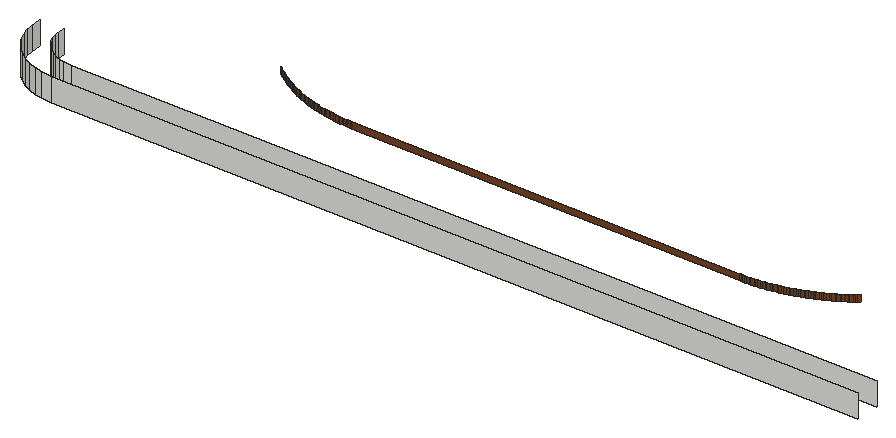
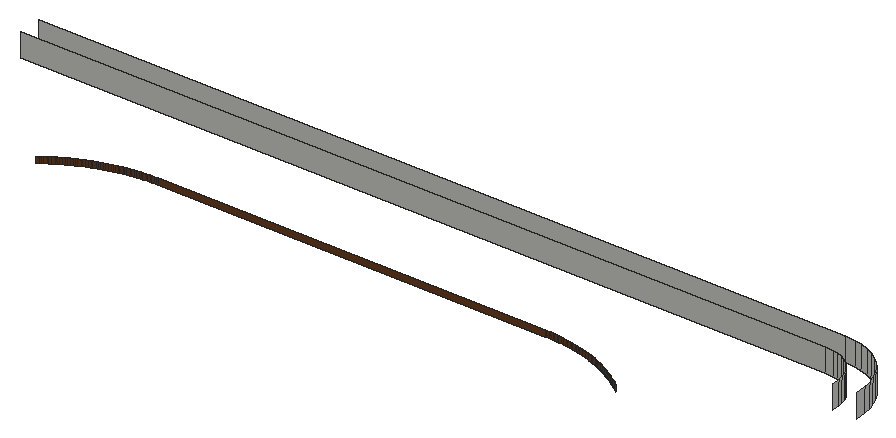
# SketchUp Ruby script. Lengths in inches.
U = 1.inch
M = Sketchup.active_model
def pt(a) = Geom::Point3d.new(a.map { |v| v * U })
def face(e, loops, mat)
  f = e.add_face(loops[0].map { |a| pt(a) })
  loops[1..].each { |l| e.add_face(l.map { |a| pt(a) }).erase! }
  f.material = f.back_material = mat if mat
  f
end
# faces: each face lists its corners as indices into pts; further lists are holes
def faces(e, pts, list, mat = nil) = list.each { |f| face(e, (f[0].is_a?(Array) ? f : [f]).map { |l| l.map { |i| pts[i] } }, mat) }
# xy, xz, yz: faces in a plane at the given z, y or x. An outline is a flat list of corners, or four numbers for a rectangle; further outlines are holes
def ring(l) = l.size == 4 ? [[l[0], l[1]], [l[2], l[1]], [l[2], l[3]], [l[0], l[3]]] : l.each_slice(2).to_a
def flat(e, list, mat, &to3) = list.each { |f| face(e, (f[0].is_a?(Array) ? f : [f]).map { |l| ring(l).map { |u, v| to3.(u, v) } }, mat) }
def xy(e, z, list, mat = nil) = flat(e, list, mat) { |x, y| [x, y, z] }
def xz(e, y, list, mat = nil) = flat(e, list, mat) { |x, z| [x, y, z] }
def yz(e, x, list, mat = nil) = flat(e, list, mat) { |y, z| [x, y, z] }
def lines(e, pts, list) = list.each { |a, b| e.add_line(pt(pts[a]), pt(pts[b])) }
# prism: a flat outline (further loops are holes) pulled along v
def prism(e, loops, v, mat = nil)
  f = face(e, loops, mat); d = Geom::Vector3d.new(v.map { |x| x * U })
  f.pushpull(f.normal.samedirection?(d) ? d.length : -d.length)
end
def box(e, o, s, mat = nil) = prism(e, [[o, [o[0] + s[0], o[1], o[2]], [o[0] + s[0], o[1] + s[1], o[2]], [o[0], o[1] + s[1], o[2]]]], [0, 0, s[2]], mat)
def at(x, y, z, deg = 0) = Geom::Transformation.translation(pt([x, y, z])) * Geom::Transformation.rotation(ORIGIN, Z_AXIS, deg.degrees)
def axes(o, x, y, z) = Geom::Transformation.new([*x, 0, *y, 0, *z, 0, *pt(o).to_a, 1])
def part(name) = M.definitions.add(name)
# library, detail: a bought-in or finely detailed component or shape, given as its bounding box
def library(name, o, s) = part(name).tap { |d| box(d.entities, o, s) }
def detail(e, o, s) = box(e.add_group.entities, o, s)
def put(e, d, t, mat = nil) = e.add_instance(d, t).tap { |i| i.material = mat if mat }
def group(e, t, mat = nil) = e.add_group.tap { |g| g.transformation = t; g.material = mat if mat }.entities
root = M.entities
M.materials.add("[Wood Veneer 01]3").color = [120, 70, 37]
xz(root,33.75,[[75.22,121,143.98,123]])
xz(root,35.75,[[75.29,121,143.97,123]])
xz(root,43.5,[[92.65,121,92.82,121.5],[92.82,121,93,121.5],[93,121,126,121.5],[126,121,126.18,121.5],[126.18,121,126.35,121.5]],"[Wood Veneer 01]3")
p = [[73.64,33.94,121],[74.32,33.81,121],[74.32,33.81,123],[73.64,33.94,123],[75.22,33.75,121],[75.22,33.75,123],
  [73,34.16,121],[73,34.16,123],[72.38,34.47,121],[72.38,34.47,123],[71.8125,34.85,121],[71.8125,34.85,123],
  [71.3,35.3,121],[71.3,35.3,123],[70.85,35.8125,121],[70.85,35.8125,123],[70.47,36.38,121],[70.47,36.38,123],
  [74.58,35.8,121],[74.16,35.88,121],[74.16,35.88,123],[74.58,35.8,123],[75.29,35.75,121],[75.29,35.75,123],
  [73.76,36.01,121],[73.76,36.01,123],[73.38,36.2,121],[73.38,36.2,123],[73.03,36.4375,121],[73.03,36.4375,123],
  [70.16,37,121],[70.16,37,123],[72.72,36.72,121],[72.72,36.72,123],[72.4375,37.03,121],[72.4375,37.03,123],
  [69.94,37.64,121],[69.94,37.64,123],[72.2,37.38,121],[72.2,37.38,123],[72.01,37.76,121],[72.01,37.76,123],
  [69.81,38.32,121],[69.81,38.32,123],[71.88,38.16,121],[71.88,38.16,123],[71.8,38.58,121],[71.8,38.58,123],
  [69.75,39.22,121],[69.75,39.22,123],[71.75,39.29,121],[71.75,39.29,123],[91.76,43.56,121],[91.94,43.54,121],
  [91.94,43.54,121.5],[91.76,43.56,121.5],[92.12,43.53,121],[92.12,43.53,121.5],[92.29,43.52,121],[92.29,43.52,121.5],
  [92.47,43.51,121],[92.47,43.51,121.5],[92.65,43.5,121],[92.65,43.5,121.5],[126.35,43.5,121],[126.53,43.51,121],
  [126.53,43.51,121.5],[126.35,43.5,121.5],[126.71,43.52,121],[126.71,43.52,121.5],[126.88,43.53,121],[126.88,43.53,121.5],
  [127.06,43.54,121],[127.06,43.54,121.5],[127.24,43.56,121],[127.24,43.56,121.5],[90.89,43.67,121],[91.0625,43.64,121],
  [91.0625,43.64,121.5],[90.89,43.67,121.5],[91.24,43.62,121],[91.24,43.62,121.5],[91.41,43.59,121],[91.41,43.59,121.5],
  [91.59,43.57,121],[91.59,43.57,121.5],[127.41,43.57,121],[127.41,43.57,121.5],[127.59,43.59,121],[127.59,43.59,121.5],
  [127.76,43.62,121],[127.76,43.62,121.5],[127.9375,43.64,121],[127.9375,43.64,121.5],[128.11,43.67,121],[128.11,43.67,121.5],
  [90.37,43.76,121],[90.54,43.73,121],[90.54,43.73,121.5],[90.37,43.76,121.5],[90.71,43.69,121],[90.71,43.69,121.5],
  [128.29,43.69,121],[128.29,43.69,121.5],[128.46,43.73,121],[128.46,43.73,121.5],[128.63,43.76,121],[128.63,43.76,121.5],
  [89.85,43.87,121],[90.02,43.83,121],[90.02,43.83,121.5],[89.85,43.87,121.5],[90.19,43.79,121],[90.19,43.79,121.5],
  [128.81,43.79,121],[128.81,43.79,121.5],[128.98,43.83,121],[128.98,43.83,121.5],[129.15,43.87,121],[129.15,43.87,121.5],
  [89.51,43.96,121],[89.68,43.92,121],[89.68,43.92,121.5],[89.51,43.96,121.5],[129.32,43.92,121],[129.32,43.92,121.5],
  [129.49,43.96,121],[129.49,43.96,121.5],[89.17,44.06,121],[89.34,44.01,121],[89.34,44.01,121.5],[89.17,44.06,121.5],
  [129.66,44.01,121],[129.66,44.01,121.5],[129.83,44.06,121],[129.83,44.06,121.5],[88.83,44.16,121],[89,44.11,121],
  [89,44.11,121.5],[88.83,44.16,121.5],[130,44.11,121],[130,44.11,121.5],[130.17,44.16,121],[130.17,44.16,121.5],
  [88.49,44.27,121],[88.66,44.22,121],[88.66,44.22,121.5],[88.49,44.27,121.5],[130.34,44.22,121],[130.34,44.22,121.5],
  [130.51,44.27,121],[130.51,44.27,121.5],[88.16,44.4,121],[88.33,44.33,121],[88.33,44.33,121.5],[88.16,44.4,121.5],
  [130.67,44.33,121],[130.67,44.33,121.5],[130.84,44.4,121],[130.84,44.4,121.5],[88,44.46,121],[88,44.46,121.5],
  [131,44.46,121],[131,44.46,121.5],[87.67,44.6,121],[87.83,44.53,121],[87.83,44.53,121.5],[87.67,44.6,121.5],
  [131.17,44.53,121],[131.17,44.53,121.5],[131.33,44.6,121],[131.33,44.6,121.5],[87.51,44.67,121],[87.51,44.67,121.5],
  [131.49,44.67,121],[131.49,44.67,121.5],[87.1875,44.82,121],[87.35,44.74,121],[87.35,44.74,121.5],[87.1875,44.82,121.5],
  [131.65,44.74,121],[131.65,44.74,121.5],[131.8125,44.82,121],[131.8125,44.82,121.5],[87.03,44.89,121],[87.03,44.89,121.5],
  [131.97,44.89,121],[131.97,44.89,121.5],[86.87,44.97,121],[86.87,44.97,121.5],[132.13,44.97,121],[132.13,44.97,121.5],
  [86.71,45.05,121],[86.71,45.05,121.5],[132.29,45.05,121],[132.29,45.05,121.5],[86.4,45.22,121],[86.56,45.14,121],
  [86.56,45.14,121.5],[86.4,45.22,121.5],[132.44,45.14,121],[132.44,45.14,121.5],[132.6,45.22,121],[132.6,45.22,121.5],
  [86.25,45.31,121],[86.25,45.31,121.5],[132.75,45.31,121],[132.75,45.31,121.5],[86.1,45.4,121],[86.1,45.4,121.5],
  [132.9,45.4,121],[132.9,45.4,121.5],[85.95,45.49,121],[85.95,45.49,121.5],[133.05,45.49,121],[133.05,45.49,121.5],
  [85.8,45.58,121],[85.8,45.58,121.5],[133.2,45.58,121],[133.2,45.58,121.5],[85.65,45.68,121],[85.65,45.68,121.5],
  [133.35,45.68,121],[133.35,45.68,121.5],[85.5,45.78,121],[85.5,45.78,121.5],[133.5,45.78,121],[133.5,45.78,121.5],
  [85.35,45.875,121],[85.35,45.875,121.5],[133.65,45.875,121],[133.65,45.875,121.5],[85.21,45.98,121],[85.21,45.98,121.5],
  [133.79,45.98,121],[133.79,45.98,121.5],[85.06,46.08,121],[85.06,46.08,121.5],[133.94,46.08,121],[133.94,46.08,121.5],
  [84.92,46.18,121],[84.92,46.18,121.5],[134.08,46.18,121],[134.08,46.18,121.5],[84.78,46.29,121],[84.78,46.29,121.5],
  [134.22,46.29,121],[134.22,46.29,121.5],[84.64,46.4,121],[84.64,46.4,121.5]]
faces(root,p,[[0,1,2,3],[1,4,5,2],[6,0,3,7],[8,6,7,9],[10,8,9,11],[12,10,11,13],[14,12,13,15],[16,14,15,17],
  [18,19,20,21],[22,18,21,23],[19,24,25,20],[24,26,27,25],[26,28,29,27],[30,16,17,31],[28,32,33,29],[32,34,35,33],
  [36,30,31,37],[34,38,39,35],[38,40,41,39],[42,36,37,43],[40,44,45,41],[44,46,47,45],[48,42,43,49],[46,50,51,47]])
faces(root,p,[[52,53,54,55],[53,56,57,54],[56,58,59,57],[58,60,61,59],[60,62,63,61],[64,65,66,67],[65,68,69,66],[68,70,71,69],
  [70,72,73,71],[72,74,75,73],[76,77,78,79],[77,80,81,78],[80,82,83,81],[82,84,85,83],[84,52,55,85],[74,86,87,75],
  [86,88,89,87],[88,90,91,89],[90,92,93,91],[92,94,95,93],[96,97,98,99],[97,100,101,98],[100,76,79,101],[94,102,103,95],
  [102,104,105,103],[104,106,107,105],[108,109,110,111],[109,112,113,110],[112,96,99,113],[106,114,115,107],[114,116,117,115],[116,118,119,117],
  [120,121,122,123],[121,108,111,122],[118,124,125,119],[124,126,127,125],[128,129,130,131],[129,120,123,130],[126,132,133,127],[132,134,135,133],
  [136,137,138,139],[137,128,131,138],[134,140,141,135],[140,142,143,141],[144,145,146,147],[145,136,139,146],[142,148,149,143],[148,150,151,149],
  [152,153,154,155],[153,144,147,154],[150,156,157,151],[156,158,159,157],[160,152,155,161],[158,162,163,159],[164,165,166,167],[165,160,161,166],
  [162,168,169,163],[168,170,171,169],[172,164,167,173],[170,174,175,171],[176,177,178,179],[177,172,173,178],[174,180,181,175],[180,182,183,181],
  [184,176,179,185],[182,186,187,183],[188,184,185,189],[186,190,191,187],[192,188,189,193],[190,194,195,191],[196,197,198,199],[197,192,193,198],
  [194,200,201,195],[200,202,203,201],[204,196,199,205],[202,206,207,203],[208,204,205,209],[206,210,211,207],[212,208,209,213],[210,214,215,211],
  [216,212,213,217],[214,218,219,215],[220,216,217,221],[218,222,223,219],[224,220,221,225],[222,226,227,223],[228,224,225,229],[226,230,231,227],
  [232,228,229,233],[230,234,235,231],[236,232,233,237],[234,238,239,235],[240,236,237,241],[238,242,243,239],[244,240,241,245],[242,246,247,243],
  [248,244,245,249]],"[Wood Veneer 01]3")
